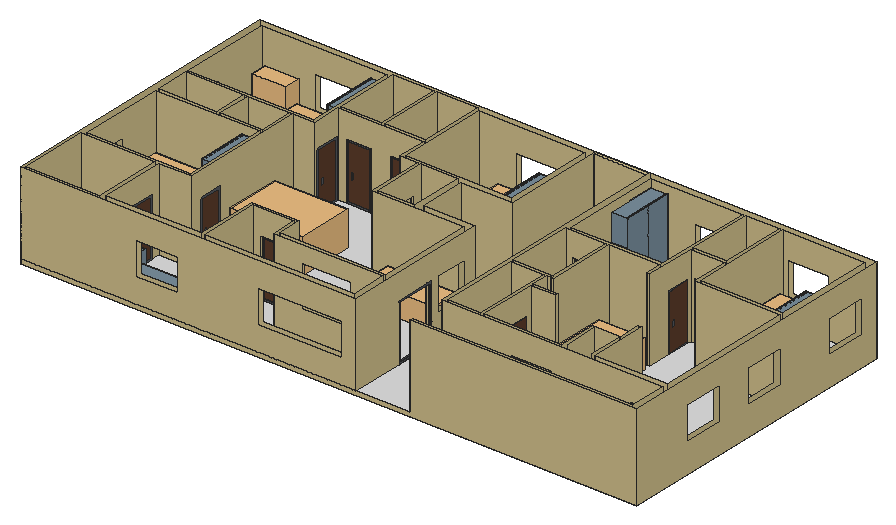
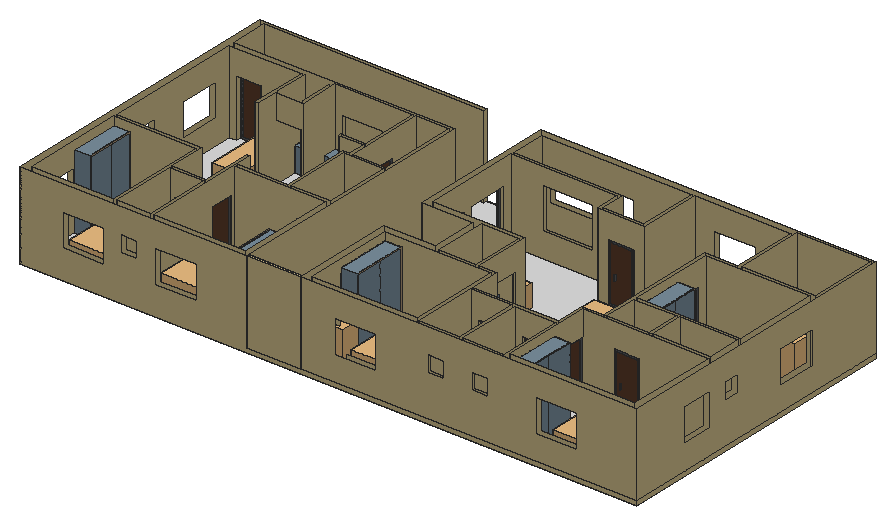
# SketchUp Ruby script. Lengths in inches.
U = 1.inch
M = Sketchup.active_model
def pt(a) = Geom::Point3d.new(a.map { |v| v * U })
def face(e, loops, mat)
  f = e.add_face(loops[0].map { |a| pt(a) })
  loops[1..].each { |l| e.add_face(l.map { |a| pt(a) }).erase! }
  f.material = f.back_material = mat if mat
  f
end
# faces: each face lists its corners as indices into pts; further lists are holes
def faces(e, pts, list, mat = nil) = list.each { |f| face(e, (f[0].is_a?(Array) ? f : [f]).map { |l| l.map { |i| pts[i] } }, mat) }
# xy, xz, yz: faces in a plane at the given z, y or x. An outline is a flat list of corners, or four numbers for a rectangle; further outlines are holes
def ring(l) = l.size == 4 ? [[l[0], l[1]], [l[2], l[1]], [l[2], l[3]], [l[0], l[3]]] : l.each_slice(2).to_a
def flat(e, list, mat, &to3) = list.each { |f| face(e, (f[0].is_a?(Array) ? f : [f]).map { |l| ring(l).map { |u, v| to3.(u, v) } }, mat) }
def xy(e, z, list, mat = nil) = flat(e, list, mat) { |x, y| [x, y, z] }
def xz(e, y, list, mat = nil) = flat(e, list, mat) { |x, z| [x, y, z] }
def yz(e, x, list, mat = nil) = flat(e, list, mat) { |y, z| [x, y, z] }
def lines(e, pts, list) = list.each { |a, b| e.add_line(pt(pts[a]), pt(pts[b])) }
# prism: a flat outline (further loops are holes) pulled along v
def prism(e, loops, v, mat = nil)
  f = face(e, loops, mat); d = Geom::Vector3d.new(v.map { |x| x * U })
  f.pushpull(f.normal.samedirection?(d) ? d.length : -d.length)
end
def box(e, o, s, mat = nil) = prism(e, [[o, [o[0] + s[0], o[1], o[2]], [o[0] + s[0], o[1] + s[1], o[2]], [o[0], o[1] + s[1], o[2]]]], [0, 0, s[2]], mat)
def at(x, y, z, deg = 0) = Geom::Transformation.translation(pt([x, y, z])) * Geom::Transformation.rotation(ORIGIN, Z_AXIS, deg.degrees)
def axes(o, x, y, z) = Geom::Transformation.new([*x, 0, *y, 0, *z, 0, *pt(o).to_a, 1])
def part(name) = M.definitions.add(name)
# library, detail: a bought-in or finely detailed component or shape, given as its bounding box
def library(name, o, s) = part(name).tap { |d| box(d.entities, o, s) }
def detail(e, o, s) = box(e.add_group.entities, o, s)
def put(e, d, t, mat = nil) = e.add_instance(d, t).tap { |i| i.material = mat if mat }
def group(e, t, mat = nil) = e.add_group.tap { |g| g.transformation = t; g.material = mat if mat }.entities
root = M.entities
M.materials.add("Flooring Laminate Dark Smoked 375cm").color = [91, 60, 43]
M.materials.add("Marble White SSS 100cm").color = [222, 222, 222]
M.materials.add("Metal Sandblasted Black 200cm").color = [86, 90, 95]
M.materials.add("Pine Highgloss 300cm").color = [174, 149, 117]
M.materials.add("Porcelain Dusk Blue Glossy 001").color = [122, 143, 157]
M.materials.add("Tiles Marble Blue 01 135cm").color = [70, 116, 149]
M.materials.add("Wall Paint Fine Grain 01 Yellow 100cm").color = [207, 190, 139]
c1 = library("Furniture Set 193 001",[-52.77,-40.82,-0.19],[105.38,81.69,50.41])
c2 = library("Ballet 2 Collar",[-24.63,-13.64,0],[49.35,27.27,70])
c3 = library("Washer 001",[-11.8125,-12.73,0],[23.63,25.47,33.9])
c4 = library("Slow",[-50.42,-21.27,0],[100.85,42.21,32.64])
c5 = library("Toilet Bowl 127 010",[-8,-12.9,0],[16,25.8,38.91])
c6 = library("Toy Table Set 40-09",[-39.37,-33.7,0],[66.93,79.21,41.36])
c7 = library("Eva Bed",[-34.4,-44.85,0.04],[68.9,90.3,39.91])
box(root,[573.63,183,0],[58.192,96.042,0.1],"Tiles Marble Blue 01 135cm")
box(root,[715.822,333,0],[49.5,96,0.1],"Tiles Marble Blue 01 135cm")
box(root,[10.815,241.5,0],[85.5,49.5,0.1],"Tiles Marble Blue 01 135cm")
box(root,[262.815,339,0.1],[60,94.5,0.1],"Tiles Marble Blue 01 135cm")
box(root,[198.315,339,0.1],[60,94.5,0.1],"Tiles Marble Blue 01 135cm")
xy(root,-6,[[1.815,1.5,898.815,438]],"Wall Paint Fine Grain 01 Yellow 100cm")
xy(root,0,[[[1.815,1.5,569.136,1.5,569.133,6,889.815,6,889.815,60,879.252,60,879.252,69,889.815,69,889.815,274.5,765.322,274.5,765.322,285,769.822,285,769.822,279,889.815,279,889.815,429,769.822,429,769.822,321,765.322,321,765.322,328.5,757.822,328.5,757.822,333,765.322,333,765.322,429,715.822,429,715.822,333,721.822,333,721.822,328.5,715.822,328.5,715.822,324.125,711.322,324.125,711.322,429,577.822,429,577.929,283.5,584.443,283.505,584.447,279.008,573.63,279,573.63,183,631.89,183,631.822,279.042,620.447,279.034,620.443,283.531,711.318,283.598,711.322,279.098,636.322,279.045,636.393,178.504,631.89,178.5,626.143,178.5,626.143,154.5,662.143,154.5,662.143,150,626.143,150,626.143,142.5,621.643,142.5,621.643,178.5,573.63,178.5,573.63,64.5,621.643,64.5,621.643,106.5,626.143,106.5,626.143,64.5,739.815,64.5,739.815,121.5,744.315,121.5,744.315,67.6875,780.315,67.6875,780.315,153,784.815,153,784.815,69,843.252,69,843.252,60,569.093,60,568.815,438,1.815,438],[415.815,217.5,490.815,286.5],[711.322,255,715.822,288.125]]],"Marble White SSS 100cm")
xy(root,0,[[631.89,178.5,636.393,178.504,636.322,279.045,711.322,279.098,711.318,283.598,620.443,283.531,620.447,279.034,631.822,279.042,631.89,183],[415.815,217.5,490.815,286.5],[415.815,217.5,490.815,286.5]],"Wall Paint Fine Grain 01 Yellow 100cm")
xy(root,0.1,[[6.315,6,114.315,6,114.315,58.5,118.815,58.5,118.815,10.5,258.315,10.5,258.315,102,274.815,102,274.815,97.5,262.815,97.5,262.815,10.5,481.815,10.5,481.815,61.5,322.815,61.5,322.815,97.5,310.815,97.5,310.815,102,327.315,102,327.315,66,481.815,66,481.815,78.6875,490.815,78.6875,490.815,138.6875,481.815,138.6875,481.815,208.5,348.315,208.5,348.315,225,352.815,225,352.815,213,406.815,213,406.815,291,352.815,291,352.815,279,348.315,279,348.315,291,322.815,291,322.815,295.5,481.815,295.5,481.815,429,327.315,429,327.315,331.5,322.815,331.5,322.815,334.5,310.815,334.5,310.815,339,322.815,339,322.815,433.5,262.815,433.5,262.815,339,274.815,339,274.815,334.5,246.315,334.5,246.315,339,258.315,339,258.315,433.5,198.315,433.5,198.315,339,210.315,339,210.315,334.5,198.315,334.5,198.315,331.5,193.815,331.5,193.815,429,10.815,429,10.815,295.5,112.03,295.5,112.03,291,100.815,291,100.815,283.5,96.315,283.5,96.315,291,10.815,291,10.815,241.5,96.315,241.5,96.315,247.5,100.815,247.5,100.815,241.5,162.315,241.5,162.315,291,148.03,291,148.03,295.5,198.315,295.5,198.315,291,166.815,291,166.815,159,162.315,159,162.315,237,10.815,237,10.815,111,162.315,111,162.315,123,166.815,123,166.815,106.5,118.815,106.5,118.815,94.5,114.315,94.5,114.315,106.5,6.315,106.5]],"Marble White SSS 100cm")
xz(root,1.5,[[1.815,-6,898.815,-6,898.815,120,569.136,120,569.136,0,1.815,0],[[1.815,0,490.815,120],[347.502,36,469.815,84],[170.627,36,230.627,84]]],"Wall Paint Fine Grain 01 Yellow 100cm")
xz(root,6,[[569.133,0,889.815,120],[6.315,0.1,114.315,120]],"Wall Paint Fine Grain 01 Yellow 100cm")
xz(root,10.5,[[[118.815,0.1,258.315,120],[170.627,36,230.627,84]],[[262.815,0.1,481.815,120],[347.502,36,469.815,84]]],"Wall Paint Fine Grain 01 Yellow 100cm")
xz(root,58.5,[[114.315,0.1,118.815,84]],"Wall Paint Fine Grain 01 Yellow 100cm")
xz(root,60,[[[569.093,0,843.252,0,843.252,84,879.252,84,879.252,0,889.815,0,889.815,120,569.093,120],[669.192,36,729.192,84]]],"Wall Paint Fine Grain 01 Yellow 100cm")
xz(root,61.5,[[[322.815,0.1,481.815,120],[363.315,36,435.315,96]]],"Wall Paint Fine Grain 01 Yellow 100cm")
xz(root,64.5,[[573.63,0,621.643,120],[626.13,0,626.143,120],[[626.143,0,739.815,120],[669.192,36,729.192,84]]],"Wall Paint Fine Grain 01 Yellow 100cm")
xz(root,66,[[[327.315,0.1,481.815,120],[363.315,36,435.315,96]]],"Wall Paint Fine Grain 01 Yellow 100cm")
xz(root,67.6875,[[744.315,0,780.315,36]],"Wall Paint Fine Grain 01 Yellow 100cm")
xz(root,69,[[784.815,0,784.815,120,889.815,120,889.815,0,879.252,0,879.252,84,843.252,84,843.252,0]],"Wall Paint Fine Grain 01 Yellow 100cm")
xz(root,78.6875,[[481.815,0.1,490.815,84]],"Wall Paint Fine Grain 01 Yellow 100cm")
xz(root,94.5,[[114.315,0.1,118.815,84]],"Wall Paint Fine Grain 01 Yellow 100cm")
xz(root,97.5,[[262.815,0.1,274.815,0.1,274.815,84,310.815,84,310.815,0.1,322.815,0.1,322.815,120,262.815,120]],"Wall Paint Fine Grain 01 Yellow 100cm")
xz(root,102,[[258.315,0.1,258.315,120,327.315,120,327.315,0.1,310.815,0.1,310.815,84,274.815,84,274.815,0.1]],"Wall Paint Fine Grain 01 Yellow 100cm")
xz(root,106.5,[[621.643,0,626.143,84],[6.315,0.1,114.315,120],[118.815,0.1,166.815,120]],"Wall Paint Fine Grain 01 Yellow 100cm")
xz(root,111,[[10.815,0.1,162.315,120]],"Wall Paint Fine Grain 01 Yellow 100cm")
xz(root,121.5,[[739.815,0,739.815,120,780.315,120,780.315,84,744.315,84,744.315,0]],"Wall Paint Fine Grain 01 Yellow 100cm")
xz(root,123,[[162.315,0.1,166.815,84]],"Wall Paint Fine Grain 01 Yellow 100cm")
xz(root,138.6875,[[481.815,0.1,490.815,84]],"Wall Paint Fine Grain 01 Yellow 100cm")
xz(root,142.5,[[621.643,0,626.143,84]],"Wall Paint Fine Grain 01 Yellow 100cm")
xz(root,150,[[626.143,0,662.143,120]],"Wall Paint Fine Grain 01 Yellow 100cm")
xz(root,153,[[780.315,0,784.815,120]],"Wall Paint Fine Grain 01 Yellow 100cm")
xz(root,154.5,[[626.143,0,662.143,120]],"Wall Paint Fine Grain 01 Yellow 100cm")
xz(root,159,[[162.315,0.1,166.815,84]],"Wall Paint Fine Grain 01 Yellow 100cm")
xz(root,178.5,[[[573.63,0,621.643,120],[584.88,60,608.88,84]],[626.143,0,631.89,120]],"Wall Paint Fine Grain 01 Yellow 100cm")
xz(root,183,[[[573.63,0,631.89,120],[584.88,60,608.88,84]]],"Wall Paint Fine Grain 01 Yellow 100cm")
xz(root,208.5,[[348.315,0.1,481.815,120]],"Wall Paint Fine Grain 01 Yellow 100cm")
xz(root,213,[[352.815,0.1,406.815,120]],"Wall Paint Fine Grain 01 Yellow 100cm")
xz(root,217.5,[[415.815,0,490.815,120]],"Wall Paint Fine Grain 01 Yellow 100cm")
xz(root,225,[[348.315,0.1,352.815,84]],"Wall Paint Fine Grain 01 Yellow 100cm")
xz(root,237,[[10.815,0.1,162.315,120]],"Wall Paint Fine Grain 01 Yellow 100cm")
xz(root,241.5,[[10.815,0.1,96.315,120],[100.815,0.1,162.315,120]],"Wall Paint Fine Grain 01 Yellow 100cm")
xz(root,247.5,[[96.315,0.1,100.815,84]],"Wall Paint Fine Grain 01 Yellow 100cm")
xz(root,255,[[711.322,0,715.822,120]],"Wall Paint Fine Grain 01 Yellow 100cm")
xz(root,274.5,[[765.322,0,889.815,120]],"Wall Paint Fine Grain 01 Yellow 100cm")
xz(root,279,[[769.822,0,889.815,120],[348.315,0.1,352.815,84]],"Wall Paint Fine Grain 01 Yellow 100cm")
xz(root,283.5,[[96.315,0.1,100.815,84]],"Wall Paint Fine Grain 01 Yellow 100cm")
xz(root,285,[[765.322,0,769.822,84]],"Wall Paint Fine Grain 01 Yellow 100cm")
xz(root,286.5,[[415.815,0,490.815,120]],"Wall Paint Fine Grain 01 Yellow 100cm")
xz(root,288.125,[[711.322,0,715.822,84]],"Wall Paint Fine Grain 01 Yellow 100cm")
xz(root,291,[[96.315,0,100.815,120],[162.315,0,166.815,120],[10.815,0.1,96.315,120],[100.815,0.1,112.03,0.1,112.03,84,148.03,84,148.03,0.1,162.315,0.1,162.315,120,100.815,120],[166.815,0.1,198.315,120],
  [322.815,0.1,348.315,120],[352.815,0.1,406.815,120]],"Wall Paint Fine Grain 01 Yellow 100cm")
xz(root,295.5,[[10.815,0.1,10.815,120,193.815,120,193.815,84,198.315,84,198.315,0.1,148.03,0.1,148.03,84,112.03,84,112.03,0.1],[322.815,0.1,322.815,84,327.315,84,327.315,120,481.815,120,481.815,0.1]],"Wall Paint Fine Grain 01 Yellow 100cm")
xz(root,321,[[765.322,0,769.822,84]],"Wall Paint Fine Grain 01 Yellow 100cm")
xz(root,324.125,[[711.322,0,715.822,84]],"Wall Paint Fine Grain 01 Yellow 100cm")
xz(root,328.5,[[715.822,0,721.822,0,721.822,84,757.822,84,757.822,0,765.322,0,765.322,120,715.822,120]],"Wall Paint Fine Grain 01 Yellow 100cm")
xz(root,331.5,[[193.815,0.1,198.315,84],[322.815,0.1,327.315,84]],"Wall Paint Fine Grain 01 Yellow 100cm")
xz(root,333,[[715.822,0,715.822,120,765.322,120,765.322,0,757.822,0,757.822,84,721.822,84,721.822,0]],"Wall Paint Fine Grain 01 Yellow 100cm")
xz(root,334.5,[[198.315,0.1,210.315,0.1,210.315,84,246.315,84,246.315,0.1,274.815,0.1,274.815,84,310.815,84,310.815,0.1,322.815,0.1,322.815,120,198.315,120]],"Wall Paint Fine Grain 01 Yellow 100cm")
xz(root,339,[[198.315,0.1,198.315,120,258.315,120,258.315,0.1,246.315,0.1,246.315,84,210.315,84,210.315,0.1],[262.815,0.1,262.815,120,322.815,120,322.815,0.1,310.815,0.1,310.815,84,274.815,84,274.815,0.1]],"Wall Paint Fine Grain 01 Yellow 100cm")
xz(root,429,[[[577.822,0,711.322,120],[642.44,36,702.44,84]],[[715.822,0,765.322,120],[728.877,60,752.877,84]],[[769.822,0,889.815,120],[777.002,36,837.002,84]],[[10.815,0.1,193.815,120],[88.19,36,148.19,84]],[[327.315,0.1,481.815,120],[381.315,36,441.315,84]]],"Wall Paint Fine Grain 01 Yellow 100cm")
xz(root,433.5,[[[198.315,0.1,258.315,120],[218.127,60,242.127,84]],[[262.815,0.1,322.815,120],[282.377,60,306.377,84]]],"Wall Paint Fine Grain 01 Yellow 100cm")
xz(root,437.875,[[[1.815,0,490.815,120],[381.315,36,441.315,84],[88.19,36,148.19,84],[282.377,60,306.377,84],[218.127,60,242.127,84]]],"Wall Paint Fine Grain 01 Yellow 100cm")
xz(root,438,[[[1.815,-6,1.815,0,568.815,0,568.815,120,898.815,120,898.815,-6],[777.002,36,837.002,84],[642.44,36,702.44,84],[728.877,60,752.877,84]]],"Wall Paint Fine Grain 01 Yellow 100cm")
yz(root,1.815,[[1.5,-6,438,0],[[1.5,0,437.875,120],[117.625,36,177.625,84],[303.6875,36,351.6875,84],[252.9375,60,276.9375,84]]],"Wall Paint Fine Grain 01 Yellow 100cm")
yz(root,6.315,[[6,0.1,106.5,120]],"Wall Paint Fine Grain 01 Yellow 100cm")
yz(root,10.815,[[[111,0.1,237,120],[117.625,36,177.625,84]],[[241.5,0.1,291,120],[252.9375,60,276.9375,84]],[[295.5,0.1,429,120],[303.6875,36,351.6875,84]]],"Wall Paint Fine Grain 01 Yellow 100cm")
yz(root,96.315,[[241.5,0.1,241.5,120,291,120,291,0.1,283.5,0.1,283.5,84,247.5,84,247.5,0.1]],"Wall Paint Fine Grain 01 Yellow 100cm")
yz(root,100.815,[[241.5,0.1,247.5,0.1,247.5,84,283.5,84,283.5,0.1,291,0.1,291,120,241.5,120]],"Wall Paint Fine Grain 01 Yellow 100cm")
yz(root,112.03,[[291,0.1,295.5,84]],"Wall Paint Fine Grain 01 Yellow 100cm")
yz(root,114.315,[[6,0.1,6,120,106.5,120,106.5,0.1,94.5,0.1,94.5,84,58.5,84,58.5,0.1]],"Wall Paint Fine Grain 01 Yellow 100cm")
yz(root,118.815,[[10.5,0.1,58.5,0.1,58.5,84,94.5,84,94.5,0.1,106.5,0.1,106.5,120,10.5,120]],"Wall Paint Fine Grain 01 Yellow 100cm")
yz(root,148.03,[[291,0.1,295.5,84]],"Wall Paint Fine Grain 01 Yellow 100cm")
yz(root,162.315,[[111,0.1,111,120,237,120,237,0.1,159,0.1,159,84,123,84,123,0.1],[241.5,0.1,291,120]],"Wall Paint Fine Grain 01 Yellow 100cm")
yz(root,166.815,[[106.5,0.1,123,0.1,123,84,159,84,159,0.1,291,0.1,291,120,106.5,120]],"Wall Paint Fine Grain 01 Yellow 100cm")
yz(root,193.815,[[331.5,0.1,331.5,84,295.5,84,295.5,120,429,120,429,0.1]],"Wall Paint Fine Grain 01 Yellow 100cm")
yz(root,198.315,[[291,0.1,295.5,0.1,295.5,84,331.5,84,331.5,0.1,334.5,0.1,334.5,120,291,120],[339,0.1,433.5,120]],"Wall Paint Fine Grain 01 Yellow 100cm")
yz(root,210.315,[[334.5,0.1,339,84]],"Wall Paint Fine Grain 01 Yellow 100cm")
yz(root,246.315,[[334.5,0.1,339,84]],"Wall Paint Fine Grain 01 Yellow 100cm")
yz(root,258.315,[[10.5,0.1,102,120],[339,0.1,433.5,120]],"Wall Paint Fine Grain 01 Yellow 100cm")
yz(root,262.815,[[10.5,0.1,97.5,120],[339,0.1,433.5,120]],"Wall Paint Fine Grain 01 Yellow 100cm")
yz(root,274.815,[[97.5,0.1,102,84],[334.5,0.1,339,84]],"Wall Paint Fine Grain 01 Yellow 100cm")
yz(root,310.815,[[97.5,0.1,102,84],[334.5,0.1,339,84]],"Wall Paint Fine Grain 01 Yellow 100cm")
yz(root,322.815,[[61.5,0.1,97.5,120],[291,0.1,291,120,334.5,120,334.5,0.1,331.5,0.1,331.5,84,295.5,84,295.5,0.1],[339,0.1,433.5,120]],"Wall Paint Fine Grain 01 Yellow 100cm")
yz(root,327.315,[[66,0.1,102,120],[331.5,0.1,429,0.1,429,120,295.5,120,295.5,84,331.5,84]],"Wall Paint Fine Grain 01 Yellow 100cm")
yz(root,348.315,[[208.5,0.1,208.5,120,291,120,291,0.1,279,0.1,279,84,225,84,225,0.1]],"Wall Paint Fine Grain 01 Yellow 100cm")
yz(root,352.815,[[213,0.1,225,0.1,225,84,279,84,279,0.1,291,0.1,291,120,213,120]],"Wall Paint Fine Grain 01 Yellow 100cm")
yz(root,406.815,[[213,0.1,291,120]],"Wall Paint Fine Grain 01 Yellow 100cm")
yz(root,415.815,[[217.5,0,286.5,120]],"Wall Paint Fine Grain 01 Yellow 100cm")
yz(root,481.815,[[10.5,0.1,61.5,120],[[66,0.1,66,120,208.5,120,208.5,0.1,138.6875,0.1,138.6875,84,78.6875,84,78.6875,0.1],[150.6875,36,198.6875,84]],[295.5,0.1,429,120]],"Wall Paint Fine Grain 01 Yellow 100cm")
yz(root,490.815,[[[1.5,0,78.6875,0,78.6875,84,138.6875,84,138.6875,0,217.5,0,217.5,120,1.5,120],[150.6875,36,198.6875,84]],[78.6875,0,138.6875,0.1],[286.5,0,437.875,120]],"Wall Paint Fine Grain 01 Yellow 100cm")
yz(root,573.63,[[64.5,0,178.5,120],[183,0,279,120]],"Wall Paint Fine Grain 01 Yellow 100cm")
yz(root,621.643,[[64.5,0,64.5,120,178.5,120,178.5,0,142.5,0,142.5,84,106.5,84,106.5,0]],"Wall Paint Fine Grain 01 Yellow 100cm")
yz(root,626.143,[[142.5,0,150,0,150,120,64.5,120,64.5,36,106.5,36,106.5,84,142.5,84],[64.5,0,106.5,36],[154.5,0,178.5,120]],"Wall Paint Fine Grain 01 Yellow 100cm")
yz(root,631.89,[[178.5,0,183,120]],"Wall Paint Fine Grain 01 Yellow 100cm")
yz(root,662.143,[[150,0,154.5,120]],"Wall Paint Fine Grain 01 Yellow 100cm")
yz(root,711.322,[[255,0,279.098,120],[279.098,0,279.098,120,429,120,429,0,324.125,0,324.125,84,288.125,84,288.125,0]],"Wall Paint Fine Grain 01 Yellow 100cm")
yz(root,715.822,[[255,0,288.125,0,288.125,84,324.125,84,324.125,0,328.5,0,328.5,120,255,120],[333,0,429,120]],"Wall Paint Fine Grain 01 Yellow 100cm")
yz(root,721.822,[[328.5,0,333,84]],"Wall Paint Fine Grain 01 Yellow 100cm")
yz(root,739.815,[[64.5,0,121.5,120]],"Wall Paint Fine Grain 01 Yellow 100cm")
yz(root,744.315,[[67.6875,0,121.5,0,121.5,84,117,84,117,120,69,120,69,36,67.6875,36]],"Wall Paint Fine Grain 01 Yellow 100cm")
yz(root,757.822,[[328.5,0,333,84]],"Wall Paint Fine Grain 01 Yellow 100cm")
yz(root,765.322,[[274.5,0,274.5,120,328.5,120,328.5,0,321,0,321,84,285,84,285,0],[333,0,429,120]],"Wall Paint Fine Grain 01 Yellow 100cm")
yz(root,769.822,[[279,0,285,0,285,84,321,84,321,0,429,0,429,120,279,120]],"Wall Paint Fine Grain 01 Yellow 100cm")
yz(root,780.315,[[67.6875,0,67.6875,36,69,36,69,120,117,120,117,84,121.5,84,121.5,120,153,120,153,0]],"Wall Paint Fine Grain 01 Yellow 100cm")
yz(root,784.815,[[69,0,153,120]],"Wall Paint Fine Grain 01 Yellow 100cm")
yz(root,843.252,[[60,0,69,84]],"Wall Paint Fine Grain 01 Yellow 100cm")
yz(root,879.252,[[60,0,69,84]],"Wall Paint Fine Grain 01 Yellow 100cm")
yz(root,889.815,[[6,0,60,120],[[69,0,274.5,120],[94,36,154,84],[203.625,36,263.625,84]],[[279,0,429,120],[351.6875,36,411.6875,84]]],"Wall Paint Fine Grain 01 Yellow 100cm")
yz(root,898.815,[[[1.5,-6,438,120],[94,36,154,84],[203.625,36,263.625,84],[351.6875,36,411.6875,84]]],"Wall Paint Fine Grain 01 Yellow 100cm")
p = [[569.133,6,120],[569.133,6,0],[569.136,1.5,0],[569.136,1.5,120],[568.815,438,0],[569.093,60,0],
  [569.093,60,120],[568.815,438,120],[636.393,178.504,120],[631.89,178.5,120],[631.89,178.5,0],[636.393,178.504,0],
  [636.322,279.045,0],[636.322,279.045,120],[636.322,279.043,120],[631.822,279.042,0],[631.89,183,0],[631.89,183,120],
  [631.822,279.042,120],[584.447,279.008,0],[584.447,279.008,84],[620.447,279.034,84],[620.447,279.034,0],[573.63,279,120],
  [573.63,279,0],[584.443,283.505,84],[584.443,283.505,0],[620.443,283.531,84],[620.443,283.531,0],[711.322,279.098,120],
  [711.322,279.098,0],[711.318,283.598,0],[711.318,283.598,120],[577.822,429,120],[577.929,283.5,120],[577.929,283.5,0],
  [577.822,429,0]]
faces(root,p,[[0,1,2,3],[4,5,6,7],[8,9,10,11],[12,13,14,8,11],[15,16,17,18],[19,20,21,22,15,18,23,24],[25,20,19,26],[27,28,22,21],
  [29,13,12,30],[30,31,32,29],[33,34,35,36],[31,28,27,25,26,35,34,32]],"Wall Paint Fine Grain 01 Yellow 100cm")
put(root,c1,at(222.92,213.74,0))
put(root,c2,at(587.16,329.32,0,90))
put(root,c2,at(457.06,421.0625,0))
put(root,c2,at(40.98,418.66,0))
put(root,c3,at(601.1875,164.8,0))
put(root,c3,at(25.13,92.61,0))
put(root,c3,at(52.5,92.34,0))
put(root,c4,at(424.06,184.22,0))
put(root,c4,at(810.94,122.36,0,90))
put(root,c5,at(23.8,263.28,0,90))
put(root,c5,at(601.81,196.24,0,180))
g1 = group(root,at(577.85,429,0),"Pine Highgloss 300cm")
xy(g1,0,[[0,-72.6875,24,0]],"Porcelain Dusk Blue Glossy 001")
xy(g1,108,[[0,-72.6875,24,0]],"Porcelain Dusk Blue Glossy 001")
xz(g1,-72.6875,[[0,0,24,108]],"Porcelain Dusk Blue Glossy 001")
xz(g1,0,[[0,0,24,108]],"Porcelain Dusk Blue Glossy 001")
yz(g1,0,[[-72.6875,0,0,108]],"Porcelain Dusk Blue Glossy 001")
yz(g1,24,[[[-72.6,0.09,-0.09,107.91],[-72.05,0.64,-0.64,107.36]]],"Pine Highgloss 300cm")
g2 = group(g1,at(24,-36.34,0.64))
box(g2,[-2.08,-35.7,0],[2.08,35.7,106.72],"Porcelain Dusk Blue Glossy 001")
g3 = group(g1,at(24,-0.64,0.64))
box(g3,[-2.08,-35.7,0],[2.08,35.7,106.72],"Porcelain Dusk Blue Glossy 001")
put(root,c2,at(35.54,125.6875,0,180))
g4 = group(root,at(382.81,213,0),"Pine Highgloss 300cm")
xy(g4,0,[[0,0,24,78]],"Pine Highgloss 300cm")
xy(g4,36,[[0,0,24,78]],"Pine Highgloss 300cm")
xz(g4,0,[[0,0,24,36]],"Pine Highgloss 300cm")
xz(g4,78,[[0,0,24,36]],"Porcelain Dusk Blue Glossy 001")
yz(g4,0,[[0,0,78,36]],"Porcelain Dusk Blue Glossy 001")
yz(g4,24,[[0,0,78,36]],"Pine Highgloss 300cm")
g5 = group(g4,at(0,39,0.71),"Porcelain Dusk Blue Glossy 001")
box(g5,[0,0,0],[0.71,38.29,34.58],"Porcelain Dusk Blue Glossy 001")
g6 = group(g4,at(0,0.71,0.71))
box(g6,[0,0,0],[0.71,38.29,34.58],"Porcelain Dusk Blue Glossy 001")
g7 = group(root,at(490.81,78.6875,0))
prism(g7,[[[0,60,0],[0,60,84],[0,0,84],[0,0,0]],[[0,2,2],[0,2,82],[0,58,82],[0,58,2]]],[-2.5,0,0],"Metal Sandblasted Black 200cm")
g8 = group(root,at(274.81,102,0))
prism(g8,[[[0,0,0],[0,0,84],[36,0,84],[36,0,0]],[[2,0,2],[34,0,2],[34,0,82],[2,0,82]]],[0,-2.5,0],"Metal Sandblasted Black 200cm")
g9 = group(g8,at(2,0,2))
box(g9,[0,-0.71,0],[32,0.71,80],"Flooring Laminate Dark Smoked 375cm")
g10 = group(g9,at(26,0,32),"Metal Sandblasted Black 200cm")
box(g10,[-1.5,0,0],[1.5,0.5,8])
g11 = group(root,at(322.81,295.5,0))
prism(g11,[[[0,0,0],[0,0,84],[0,36,84],[0,36,0]],[[0,34,82],[0,2,82],[0,2,2],[0,34,2]]],[2.5,0,0],"Metal Sandblasted Black 200cm")
g12 = group(g11,at(0,2,2))
box(g12,[0,0,0],[0.71,32,80],"Flooring Laminate Dark Smoked 375cm")
g13 = group(g12,at(0,26,32))
box(g13,[-0.5,-1.5,0],[0.5,1.5,8],"Metal Sandblasted Black 200cm")
g14 = group(root,at(274.81,334.5,0))
prism(g14,[[[36,0,0],[36,0,84],[0,0,84],[0,0,0]],[[34,0,2],[2,0,2],[2,0,82],[34,0,82]]],[0,2.5,0],"Metal Sandblasted Black 200cm")
g15 = group(g14,at(2,0,2))
box(g15,[0,0,0],[32,0.71,80],"Flooring Laminate Dark Smoked 375cm")
g16 = group(g15,at(6,0,32),"Metal Sandblasted Black 200cm")
xy(g16,0,[[0,-0.5,1.5,0]])
xy(g16,8,[[0,-0.5,1.5,0]])
xz(g16,-0.5,[[0,0,1.5,8]],"Metal Sandblasted Black 200cm")
xz(g16,0,[[0,0,1.5,8]],"Metal Sandblasted Black 200cm")
yz(g16,0,[[-0.5,0,0,8]])
yz(g16,1.5,[[-0.5,0,0,8]])
g17 = group(root,at(210.31,334.5,0))
prism(g17,[[[36,0,0],[36,0,84],[0,0,84],[0,0,0]],[[34,0,2],[2,0,2],[2,0,82],[34,0,82]]],[0,2.5,0],"Metal Sandblasted Black 200cm")
g18 = group(g17,at(2,0,2))
box(g18,[0,0,0],[32,0.71,80],"Flooring Laminate Dark Smoked 375cm")
g19 = group(g18,at(6,0,32),"Metal Sandblasted Black 200cm")
xy(g19,0,[[0,-0.5,1.5,0]])
xy(g19,8,[[0,-0.5,1.5,0]])
xz(g19,-0.5,[[0,0,1.5,8]],"Metal Sandblasted Black 200cm")
xz(g19,0,[[0,0,1.5,8]],"Metal Sandblasted Black 200cm")
yz(g19,0,[[-0.5,0,0,8]])
yz(g19,1.5,[[-0.5,0,0,8]])
g20 = group(root,at(198.31,295.5,0))
prism(g20,[[[0,36,0],[0,36,84],[0,0,84],[0,0,0]],[[0,34,82],[0,34,2],[0,2,2],[0,2,82]]],[-2.5,0,0],"Metal Sandblasted Black 200cm")
g21 = group(g20,at(0,2,2))
box(g21,[-0.71,0,0],[0.71,32,80],"Flooring Laminate Dark Smoked 375cm")
g22 = group(g21,at(0,6,32),"Metal Sandblasted Black 200cm")
box(g22,[0,0,0],[0.5,1.5,8])
g23 = group(root,at(166.81,123,0))
prism(g23,[[[0,36,0],[0,36,84],[0,0,84],[0,0,0]],[[0,34,2],[0,2,2],[0,2,82],[0,34,82]]],[-2.5,0,0],"Metal Sandblasted Black 200cm")
g24 = group(g23,at(0,2,2))
box(g24,[-0.71,0,0],[0.71,32,80],"Flooring Laminate Dark Smoked 375cm")
g25 = group(g24,at(0,6,32),"Metal Sandblasted Black 200cm")
box(g25,[0,0,0],[0.5,1.5,8])
g26 = group(root,at(118.81,58.5,0))
prism(g26,[[[0,36,0],[0,36,84],[0,0,84],[0,0,0]],[[0,34,2],[0,2,2],[0,2,82],[0,34,82]]],[-2.5,0,0],"Metal Sandblasted Black 200cm")
g27 = group(g26,at(0,2,2))
box(g27,[-0.71,0,0],[0.71,32,80],"Flooring Laminate Dark Smoked 375cm")
g28 = group(g27,at(0,6,32),"Metal Sandblasted Black 200cm")
box(g28,[0,0,0],[0.5,1.5,8])
g29 = group(root,at(100.81,247.5,0))
prism(g29,[[[0,36,0],[0,36,84],[0,0,84],[0,0,0]],[[0,34,2],[0,2,2],[0,2,82],[0,34,82]]],[-2.5,0,0],"Metal Sandblasted Black 200cm")
g30 = group(g29,at(0,2,2))
box(g30,[-0.71,0,0],[0.71,32,80],"Flooring Laminate Dark Smoked 375cm")
g31 = group(g30,at(0,6,32))
box(g31,[0,0,0],[0.5,1.5,8],"Metal Sandblasted Black 200cm")
g32 = group(root,at(112.03,295.5,0))
prism(g32,[[[0,0,0],[0,0,84],[36,0,84],[36,0,0]],[[34,0,82],[2,0,82],[2,0,2],[34,0,2]]],[0,-2.5,0],"Metal Sandblasted Black 200cm")
g33 = group(g32,at(2,0,2))
box(g33,[0,-0.71,0],[32,0.71,80],"Flooring Laminate Dark Smoked 375cm")
g34 = group(g33,at(26,0,32),"Metal Sandblasted Black 200cm")
box(g34,[-1.5,0,0],[1.5,0.5,8])
g35 = group(root,at(626.14,64.5,0),"Porcelain Dusk Blue Glossy 001")
prism(g35,[[[113.67,20,0],[113.67,0,0],[0,0,0],[0,42,0],[20,42,0],[20,20,0]]],[0,0,36],"Porcelain Dusk Blue Glossy 001")
g36 = group(root,at(744.31,69,0),"Porcelain Dusk Blue Glossy 001")
box(g36,[0,0,0],[36,18,36],"Porcelain Dusk Blue Glossy 001")
g37 = group(root,at(626.14,106.5,0))
prism(g37,[[[0,36,0],[0,36,84],[0,0,84],[0,0,0]],[[0,2,82],[0,34,82],[0,34,2],[0,2,2]]],[-2.5,0,0],"Metal Sandblasted Black 200cm")
g38 = group(g37,at(0,2,2))
box(g38,[-0.71,0,0],[0.71,32,80],"Flooring Laminate Dark Smoked 375cm")
g39 = group(g38,at(0,6,32),"Metal Sandblasted Black 200cm")
box(g39,[0,0,0],[0.5,1.5,8])
g40 = group(root,at(715.82,288.125,0))
prism(g40,[[[0,36,0],[0,36,84],[0,0,84],[0,0,0]],[[0,2,82],[0,34,82],[0,34,2],[0,2,2]]],[-2.5,0,0],"Metal Sandblasted Black 200cm")
g41 = group(g40,at(0,2,2))
box(g41,[-0.71,0,0],[0.71,32,80],"Flooring Laminate Dark Smoked 375cm")
g42 = group(g41,at(0,6,32),"Metal Sandblasted Black 200cm")
box(g42,[0,0,0],[0.5,1.5,8])
g43 = group(root,at(765.32,285,0))
prism(g43,[[[0,36,0],[0,0,0],[0,0,84],[0,36,84]],[[0,34,82],[0,2,82],[0,2,2],[0,34,2]]],[2.5,0,0],"Metal Sandblasted Black 200cm")
g44 = group(g43,at(0,2,2))
box(g44,[0,0,0],[0.71,32,80],"Flooring Laminate Dark Smoked 375cm")
g45 = group(g44,at(0,26,32),"Metal Sandblasted Black 200cm")
xy(g45,0,[[-0.5,-1.5,0,0]])
xy(g45,8,[[-0.5,-1.5,0,0]])
xz(g45,-1.5,[[-0.5,0,0,8]])
xz(g45,0,[[-0.5,0,0,8]])
yz(g45,-0.5,[[-1.5,0,0,8]],"Metal Sandblasted Black 200cm")
yz(g45,0,[[-1.5,0,0,8]],"Metal Sandblasted Black 200cm")
g46 = group(root,at(843.25,60,0))
prism(g46,[[[36,0,0],[36,0,84],[0,0,84],[0,0,0]],[[2,0,82],[34,0,82],[34,0,2],[2,0,2]]],[0,2.5,0],"Metal Sandblasted Black 200cm")
g47 = group(g46,at(2,0,2))
box(g47,[0,0,0],[32,0.71,80],"Flooring Laminate Dark Smoked 375cm")
g48 = group(g47,at(6,0,32),"Metal Sandblasted Black 200cm")
box(g48,[0,-0.5,0],[1.5,0.5,8])
g49 = group(root,at(721.82,328.5,0))
prism(g49,[[[0,0,0],[36,0,0],[36,0,84],[0,0,84]],[[2,0,82],[34,0,82],[34,0,2],[2,0,2]]],[0,2.5,0],"Metal Sandblasted Black 200cm")
g50 = group(g49,at(2,0,2))
box(g50,[0,0,0],[32,0.71,80],"Flooring Laminate Dark Smoked 375cm")
g51 = group(g50,at(6,0,32),"Metal Sandblasted Black 200cm")
box(g51,[0,-0.5,0],[1.5,0.5,8])
g52 = group(root,at(584.44,283.5,0))
prism(g52,[[[36,0.03,0],[0,0,0],[0,0,84],[36,0.03,84]],[[2,0,82],[2,0,2],[34,0.03,2],[34,0.03,82]]],[0,-2.5,0],"Metal Sandblasted Black 200cm")
g53 = group(g52,at(2,0,2))
prism(g53,[[[0,0,0],[32,0.02,0],[32,-0.69,0],[0,-0.71,0]]],[0,0,80],"Flooring Laminate Dark Smoked 375cm")
g54 = group(g53,at(24.5,0.02,32),"Metal Sandblasted Black 200cm")
box(g54,[0,0,0],[1.5,0.5,8])
g55 = group(root,at(490.81,325.5,0))
box(g55,[0,0,0],[39,9,8],"Marble White SSS 100cm")
g56 = group(g55,at(36.5,3.5,8),"Metal Sandblasted Black 200cm")
xy(g56,0,[[1,0,0.74,0.03,0.5,0.13,0.29,0.29,0.13,0.5,0.03,0.74,0,1,0.03,1.26,0.13,1.5,0.29,1.71,0.5,1.87,0.74,1.97,1,2,1.26,1.97,1.5,1.87,1.71,1.71,1.87,1.5,1.97,1.26,2,1,1.97,0.74,1.87,0.5,1.71,0.29,1.5,0.13,1.26,0.03]])
xy(g56,36,[[1,0,1.26,0.03,1.5,0.13,1.71,0.29,1.87,0.5,1.97,0.74,2,1,1.97,1.26,1.87,1.5,1.71,1.71,1.5,1.87,1.26,1.97,1,2,0.74,1.97,0.5,1.87,0.29,1.71,0.13,1.5,0.03,1.26,0,1,0.03,0.74,0.13,0.5,0.29,0.29,0.5,0.13,0.74,0.03]])
p = [[0.5,0.13,0],[0.74,0.03,0],[0.74,0.03,36],[0.5,0.13,36],[1,0,0],[1,0,36],
  [1.26,0.03,0],[1.26,0.03,36],[1.5,0.13,0],[1.5,0.13,36],[0.29,0.29,0],[0.29,0.29,36],
  [1.71,0.29,0],[1.71,0.29,36],[0.13,0.5,0],[0.13,0.5,36],[1.87,0.5,0],[1.87,0.5,36],
  [0.03,0.74,0],[0.03,0.74,36],[1.97,0.74,0],[1.97,0.74,36],[0,1,0],[0,1,36],
  [2,1,0],[2,1,36],[0.03,1.26,0],[0.03,1.26,36],[1.97,1.26,0],[1.97,1.26,36],
  [0.13,1.5,0],[0.13,1.5,36],[1.87,1.5,0],[1.87,1.5,36],[0.29,1.71,0],[0.29,1.71,36],
  [1.71,1.71,0],[1.71,1.71,36],[0.5,1.87,0],[0.5,1.87,36],[1.5,1.87,0],[1.5,1.87,36],
  [0.74,1.97,0],[0.74,1.97,36],[1.26,1.97,0],[1.26,1.97,36],[1,2,0],[1,2,36]]
faces(g56,p,[[0,1,2,3],[1,4,5,2],[4,6,7,5],[6,8,9,7],[10,0,3,11],[8,12,13,9],[14,10,11,15],[12,16,17,13],
  [18,14,15,19],[16,20,21,17],[22,18,19,23],[20,24,25,21],[26,22,23,27],[24,28,29,25],[30,26,27,31],[28,32,33,29],
  [34,30,31,35],[32,36,37,33],[38,34,35,39],[36,40,41,37],[42,38,39,43],[40,44,45,41],[46,42,43,47],[44,46,47,45]],"Metal Sandblasted Black 200cm")
g57 = group(root,at(490.81,433.44,0),"Wall Paint Fine Grain 01 Yellow 100cm")
prism(g57,[[[78,4.61,0],[78,0.06,0],[0,0,0],[0,4.56,0]]],[0,0,120],"Wall Paint Fine Grain 01 Yellow 100cm")
g58 = group(root,at(481.81,295.5,0),"Porcelain Dusk Blue Glossy 001")
xy(g58,0,[[-24,0,0,80.38]],"Porcelain Dusk Blue Glossy 001")
xy(g58,108,[[-24,0,0,80.38]],"Porcelain Dusk Blue Glossy 001")
xz(g58,0,[[-24,0,0,108]],"Porcelain Dusk Blue Glossy 001")
xz(g58,80.38,[[-24,0,0,108]],"Porcelain Dusk Blue Glossy 001")
yz(g58,-24,[[[0.1,0.09,80.28,107.91],[0.71,0.64,79.67,107.36]]],"Pine Highgloss 300cm")
yz(g58,0,[[0,0,80.38,108]],"Porcelain Dusk Blue Glossy 001")
g59 = group(g58,at(-24,40.1875,0.64))
box(g59,[0,0,0],[2.08,39.48,106.72],"Porcelain Dusk Blue Glossy 001")
g60 = group(g58,at(-24,0.71,0.64))
box(g60,[0,0,0],[2.08,39.48,106.72],"Porcelain Dusk Blue Glossy 001")
g61 = group(root,at(193.81,348.62,0),"Tiles Marble Blue 01 135cm")
xy(g61,0,[[-24,0,0,80.38]],"Porcelain Dusk Blue Glossy 001")
xy(g61,108,[[-24,0,0,80.38]],"Porcelain Dusk Blue Glossy 001")
xz(g61,0,[[-24,0,0,108]],"Porcelain Dusk Blue Glossy 001")
xz(g61,80.38,[[-24,0,0,108]],"Porcelain Dusk Blue Glossy 001")
yz(g61,-24,[[[0.1,0.09,80.28,107.91],[0.71,0.64,79.67,107.36]]],"Pine Highgloss 300cm")
yz(g61,0,[[0,0,80.38,108]],"Porcelain Dusk Blue Glossy 001")
g62 = group(g61,at(-24,40.1875,0.64))
box(g62,[0,0,0],[2.08,39.48,106.72],"Porcelain Dusk Blue Glossy 001")
g63 = group(g61,at(-24,0.71,0.64))
box(g63,[0,0,0],[2.08,39.48,106.72],"Porcelain Dusk Blue Glossy 001")
g64 = group(root,at(889.81,279,0),"Porcelain Dusk Blue Glossy 001")
xy(g64,0,[[-24,0,0,72.6875]],"Porcelain Dusk Blue Glossy 001")
xy(g64,108,[[-24,0,0,72.6875]],"Porcelain Dusk Blue Glossy 001")
xz(g64,0,[[-24,0,0,108]],"Porcelain Dusk Blue Glossy 001")
xz(g64,72.6875,[[-24,0,0,108]],"Porcelain Dusk Blue Glossy 001")
yz(g64,-24,[[[0.09,0.09,72.6,107.91],[0.64,0.64,72.05,107.36]]],"Pine Highgloss 300cm")
yz(g64,0,[[0,0,72.6875,108]],"Porcelain Dusk Blue Glossy 001")
g65 = group(g64,at(-24,36.34,0.64),"Porcelain Dusk Blue Glossy 001")
box(g65,[0,0,0],[2.08,35.7,106.72],"Porcelain Dusk Blue Glossy 001")
g66 = group(g64,at(-24,0.64,0.64),"Porcelain Dusk Blue Glossy 001")
box(g66,[0,0,0],[2.08,35.7,106.72],"Porcelain Dusk Blue Glossy 001")
g67 = group(root,at(162.31,162.0625,0),"Tiles Marble Blue 01 135cm")
xy(g67,0,[[-25.08,0,0,73.53]],"Porcelain Dusk Blue Glossy 001")
xy(g67,108,[[-25.08,0,0,73.53]],"Porcelain Dusk Blue Glossy 001")
xz(g67,0,[[-25.08,0,0,108]],"Porcelain Dusk Blue Glossy 001")
xz(g67,73.53,[[-25.08,0,0,108]],"Porcelain Dusk Blue Glossy 001")
yz(g67,-25.08,[[[0.09,0.09,73.44,107.91],[0.65,0.64,72.88,107.36]]],"Pine Highgloss 300cm")
yz(g67,0,[[0,0,73.53,108]],"Porcelain Dusk Blue Glossy 001")
g68 = group(g67,at(-25.08,36.76,0.64))
box(g68,[0,0,0],[2.18,36.12,106.72],"Porcelain Dusk Blue Glossy 001")
g69 = group(g67,at(-25.08,0.65,0.64))
box(g69,[0,0,0],[2.18,36.12,106.72],"Porcelain Dusk Blue Glossy 001")
g70 = group(root,at(118.81,10.5,0),"Porcelain Dusk Blue Glossy 001")
prism(g70,[[[139.5,20,0],[139.5,0,0],[0,0,0],[0,48,0],[20,48,0],[20,20,0]]],[0,0,36],"Porcelain Dusk Blue Glossy 001")
put(root,c5,at(229.43,420.7,0))
put(root,c5,at(295.09,420.6,0))
put(root,c5,at(743.9375,415.58,0))
put(root,c6,at(688.62,200.17,0))
put(root,c7,at(55.49,200.6,0,90))
put(root,c7,at(804.72,378.23,0))
put(root,c7,at(675.5,372.91,0))
put(root,c7,at(395.47,376.6,0))
put(root,c7,at(100.4375,378.82,0))
